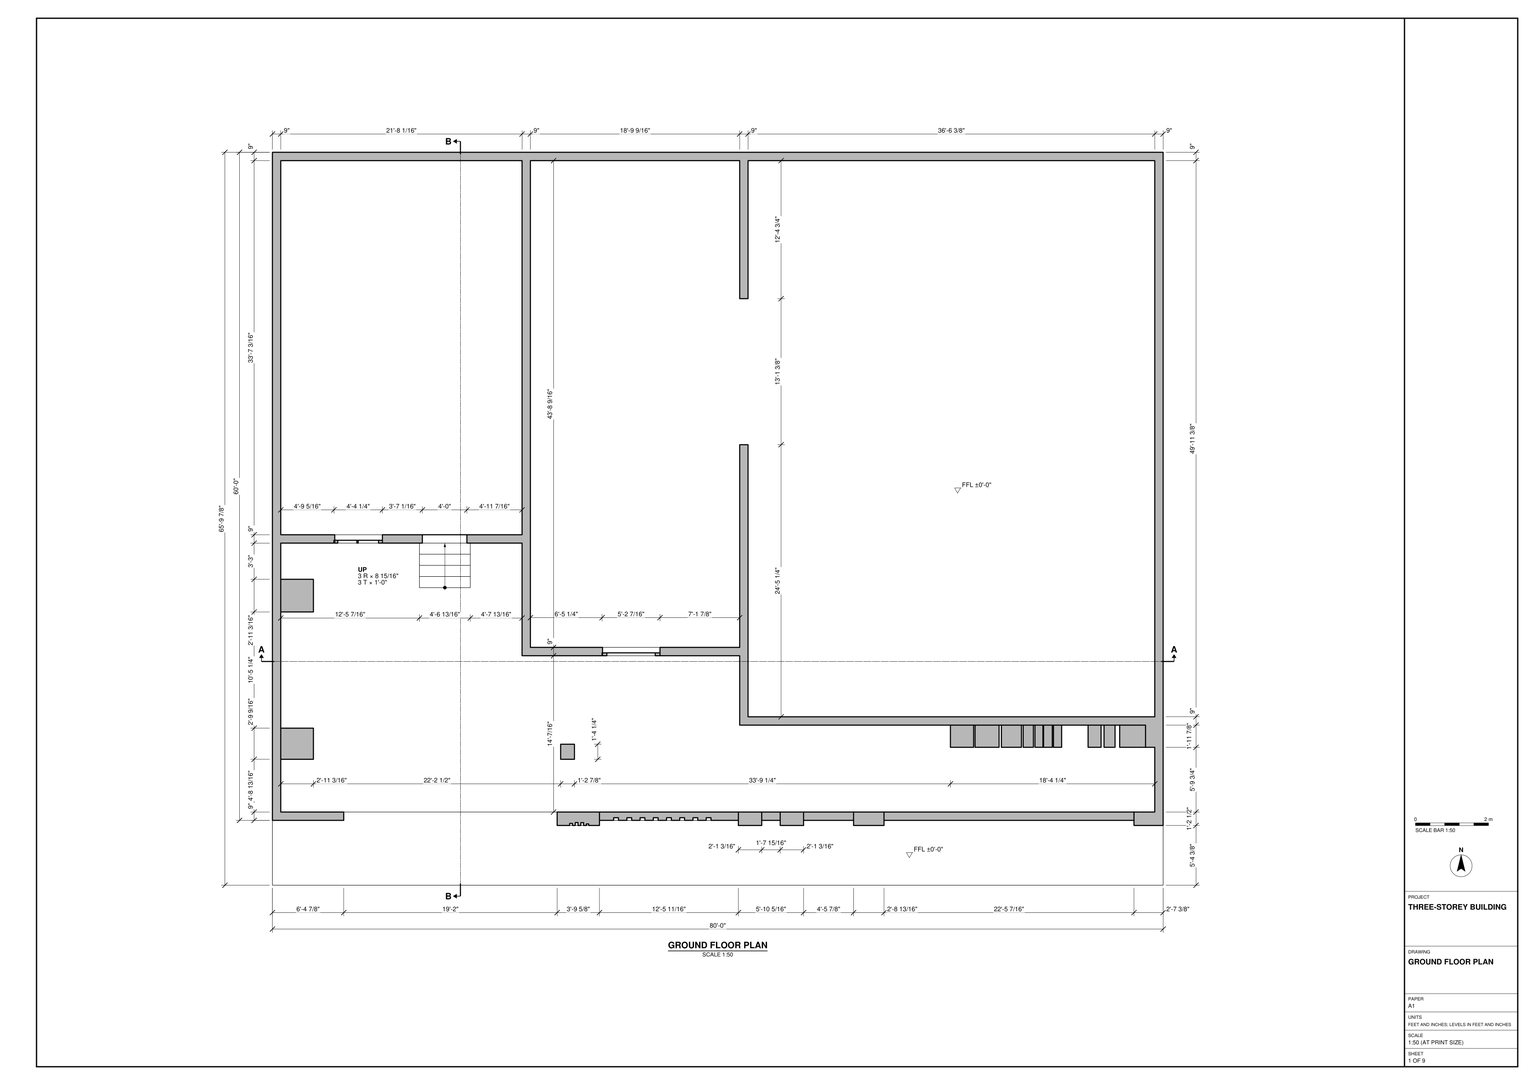
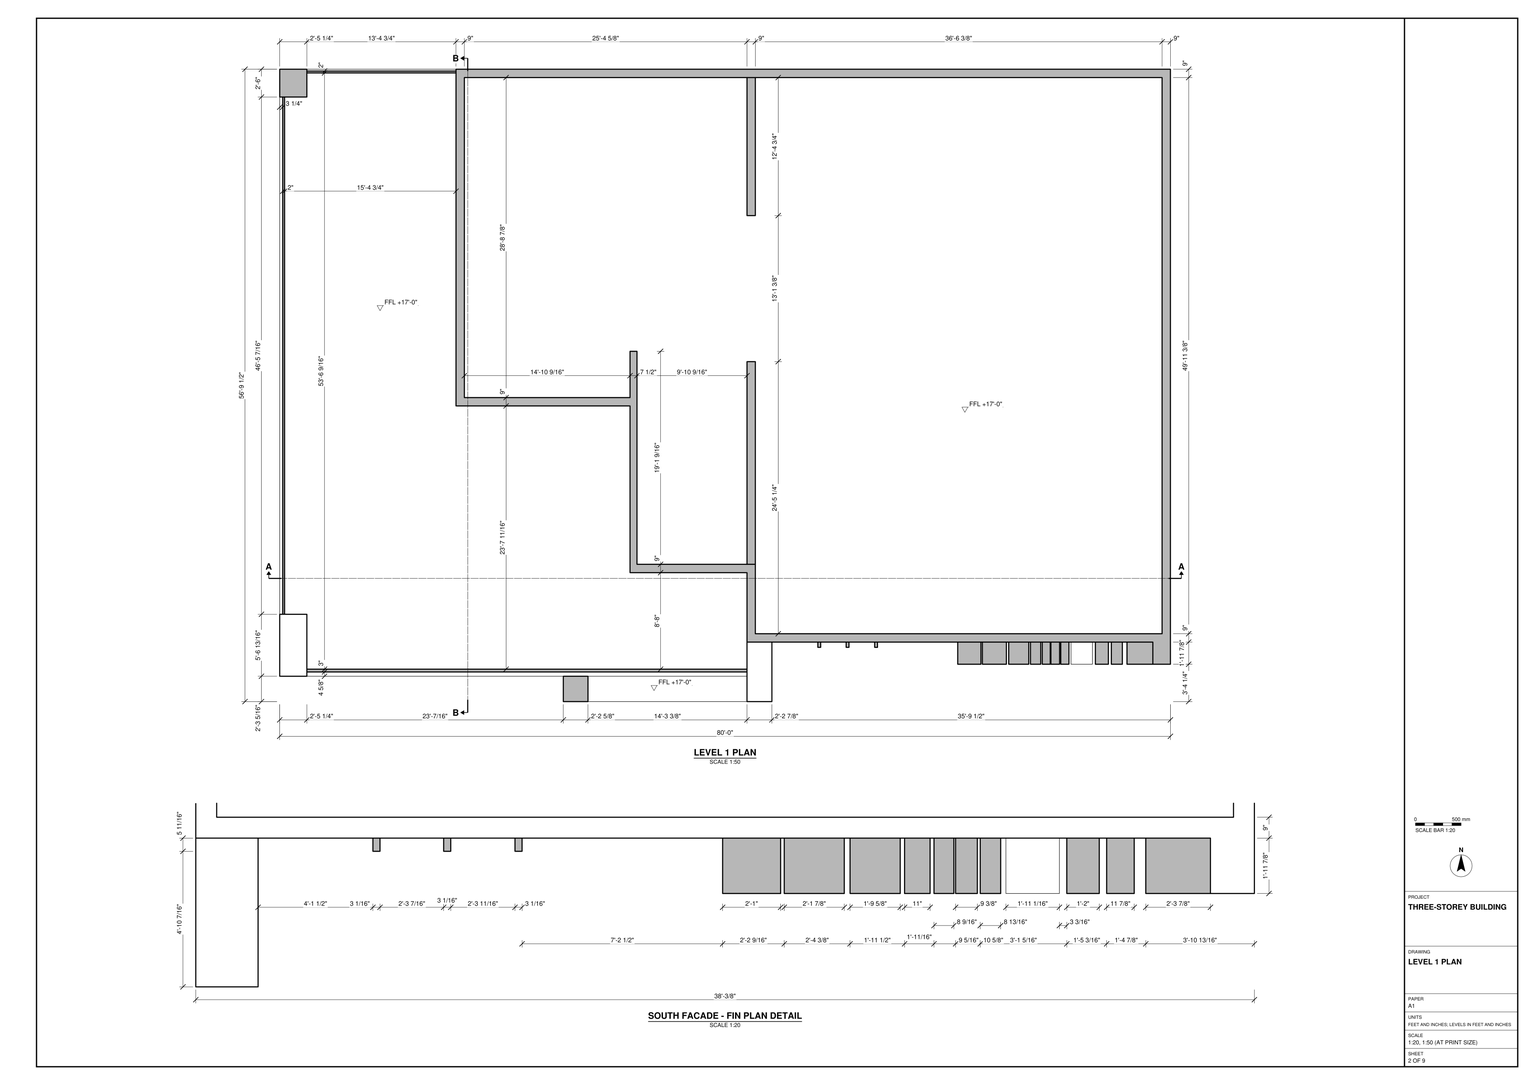
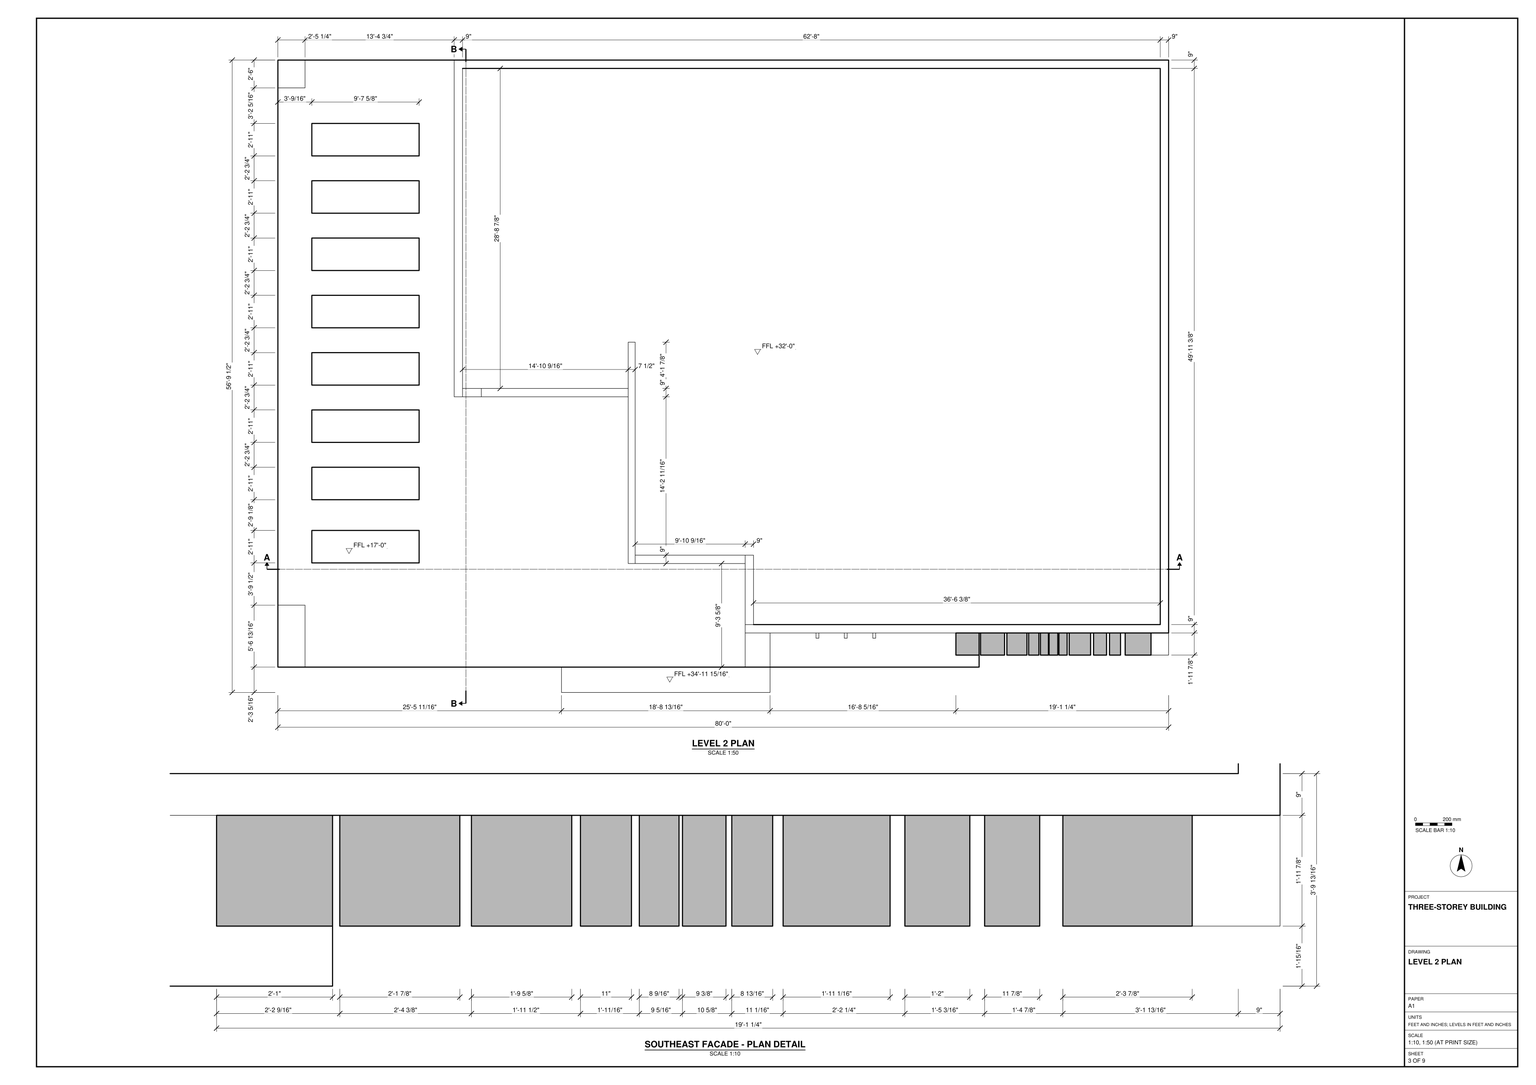
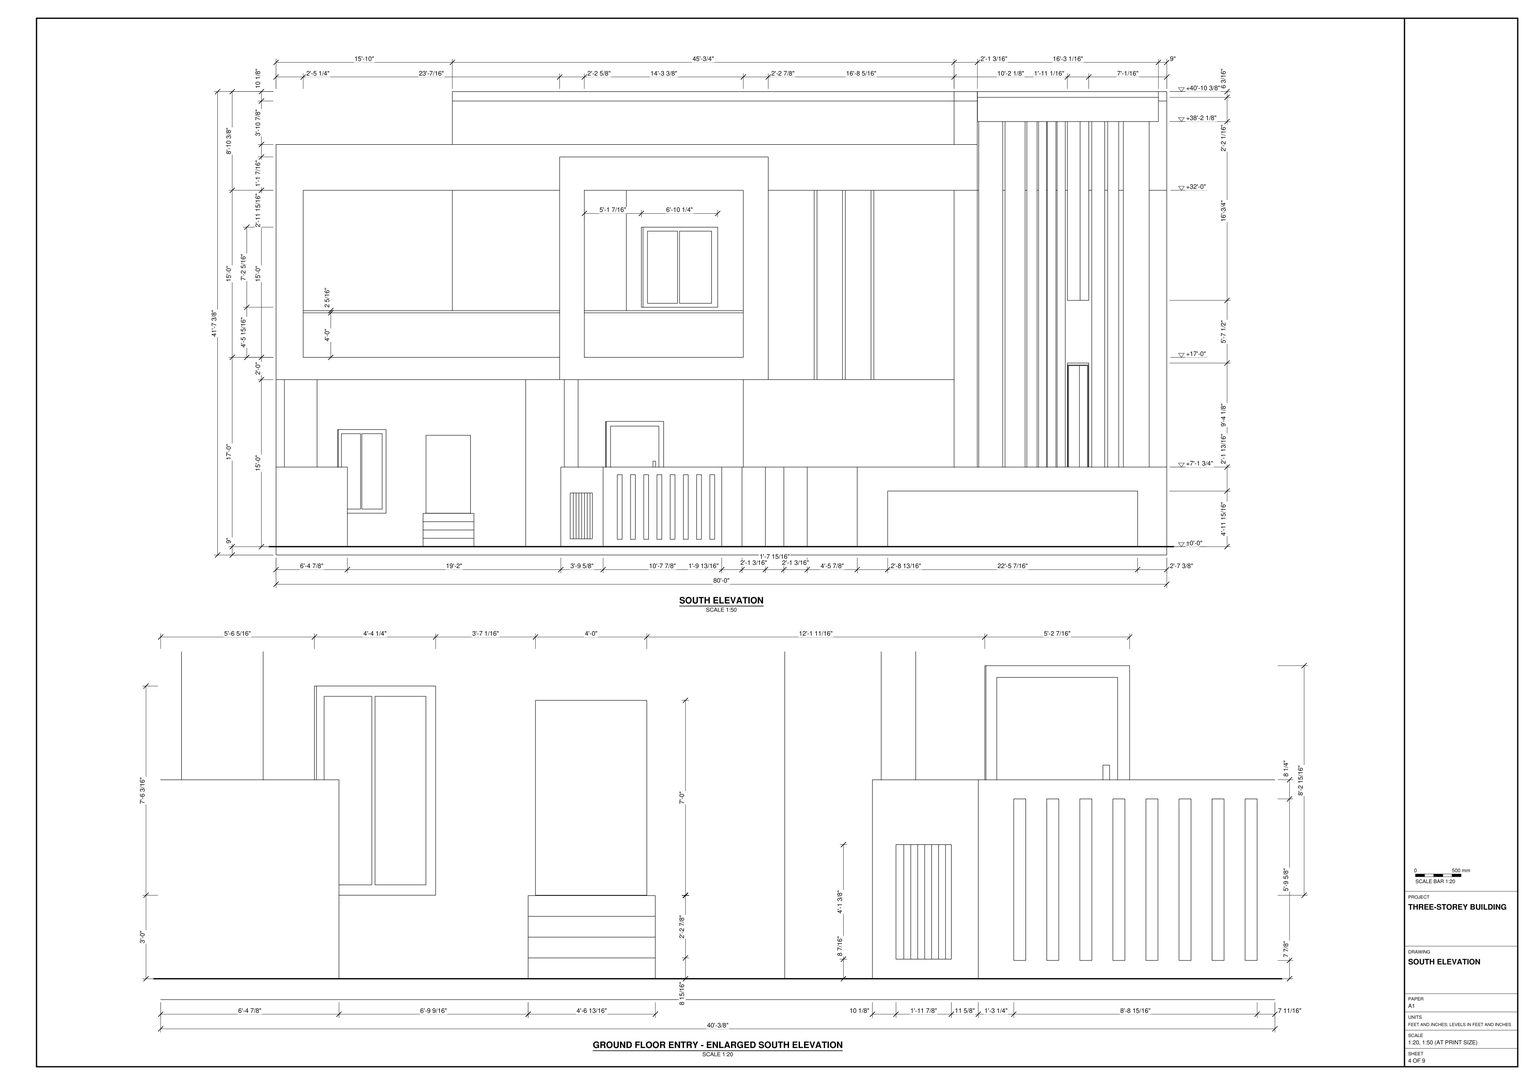
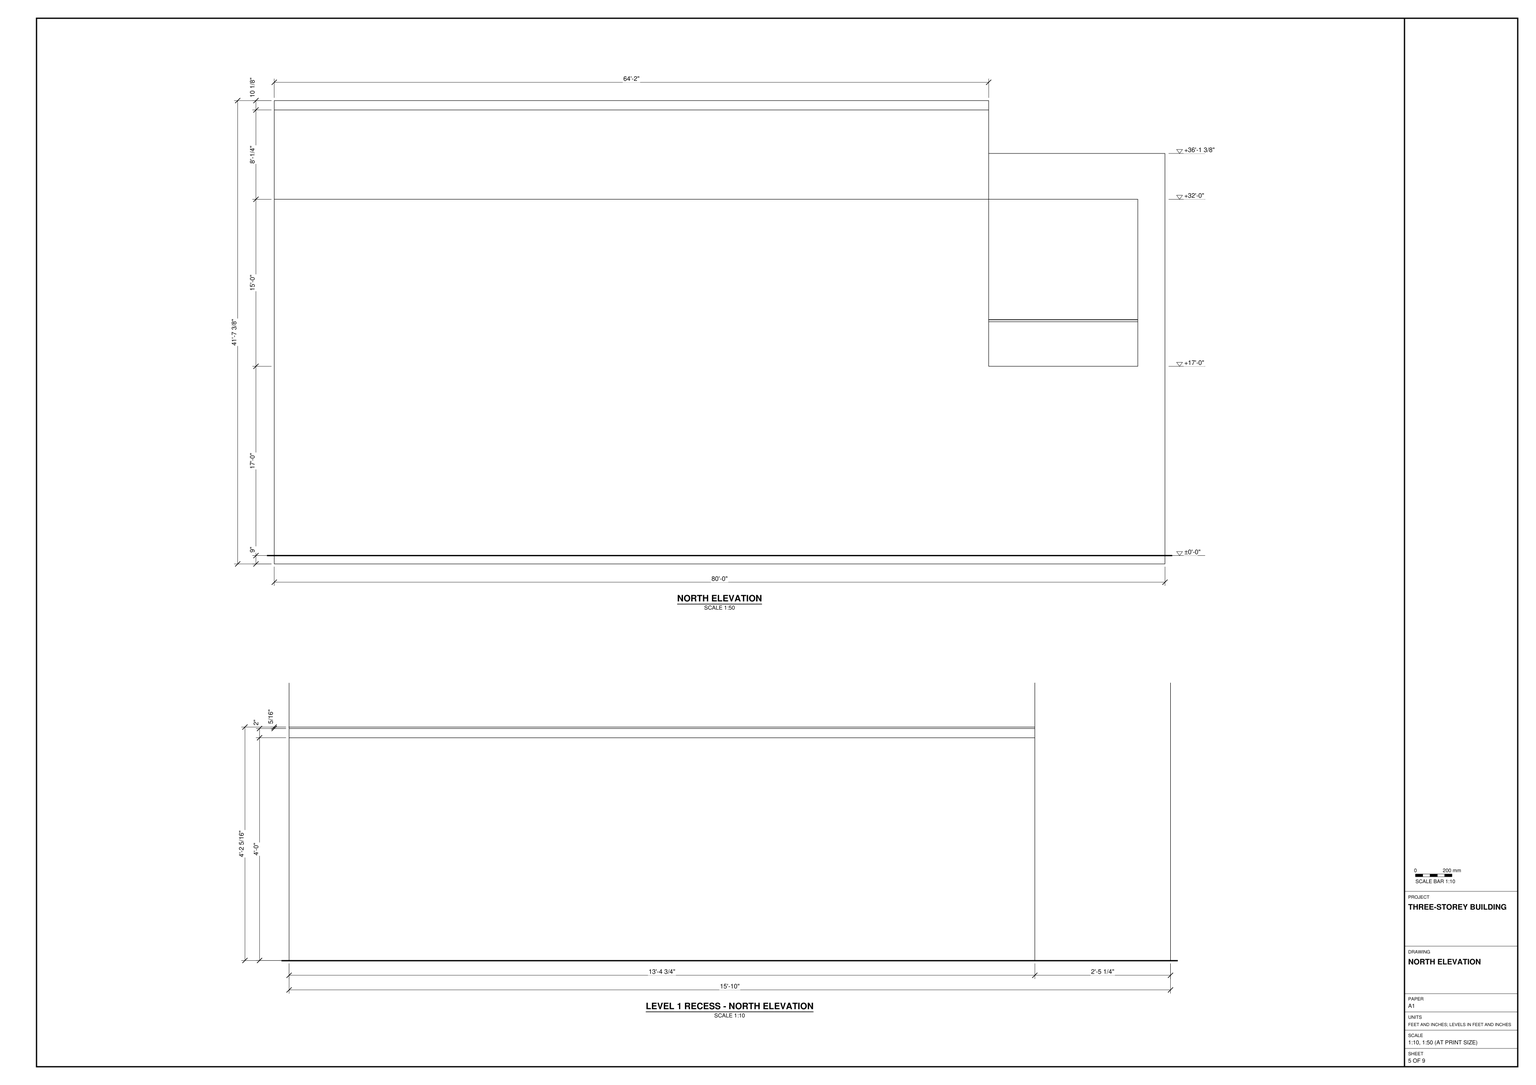
Build the three-storey building in SketchUp using task_files/diagram_01.pdf. Work in feet and inches. The overall model extents are 80'-0" east to west, 65'-9 7/8" north to south and 41'-7 3/8" vertically. Set the finished floor levels at ±0'-0", +17'-0" and +32'-0".

Lay out the ground floor from the north wall. The west, middle and east bays extend successively farther south, leaving an open area between the rooms and the south boundary wall. Follow the wall thicknesses shown, including the 9" walls. Form the door and window openings, the short stair at the south wall of the west room, and the wide entrance gap in the south boundary wall.

Follow each upper plan separately when modelling the walls, slabs and roof. Preserve the stepped enclosure and the terrace along its west and south sides. Use the upper plan to locate the row of rectangular openings above the west side. Model the projecting fins on the south face of the east bay, using the enlarged details for their widths and spacing.

Keep walls, slabs, roof, stairs and any furniture or joinery pieces shown in separate groups or components. Use components for repeated parts. Any decor or loose items shown may use suitable library components. Save one SketchUp model as output_files/three_storey_building_with_stepped_bays_and_facade_fins.skp.

# SketchUp Ruby script. Lengths in inches.
U = 1.inch
M = Sketchup.active_model
def pt(a) = Geom::Point3d.new(a.map { |v| v * U })
def face(e, loops, mat)
  f = e.add_face(loops[0].map { |a| pt(a) })
  loops[1..].each { |l| e.add_face(l.map { |a| pt(a) }).erase! }
  f.material = f.back_material = mat if mat
  f
end
# faces: each face lists its corners as indices into pts; further lists are holes
def faces(e, pts, list, mat = nil) = list.each { |f| face(e, (f[0].is_a?(Array) ? f : [f]).map { |l| l.map { |i| pts[i] } }, mat) }
# xy, xz, yz: faces in a plane at the given z, y or x. An outline is a flat list of corners, or four numbers for a rectangle; further outlines are holes
def ring(l) = l.size == 4 ? [[l[0], l[1]], [l[2], l[1]], [l[2], l[3]], [l[0], l[3]]] : l.each_slice(2).to_a
def flat(e, list, mat, &to3) = list.each { |f| face(e, (f[0].is_a?(Array) ? f : [f]).map { |l| ring(l).map { |u, v| to3.(u, v) } }, mat) }
def xy(e, z, list, mat = nil) = flat(e, list, mat) { |x, y| [x, y, z] }
def xz(e, y, list, mat = nil) = flat(e, list, mat) { |x, z| [x, y, z] }
def yz(e, x, list, mat = nil) = flat(e, list, mat) { |y, z| [x, y, z] }
def lines(e, pts, list) = list.each { |a, b| e.add_line(pt(pts[a]), pt(pts[b])) }
# prism: a flat outline (further loops are holes) pulled along v
def prism(e, loops, v, mat = nil)
  f = face(e, loops, mat); d = Geom::Vector3d.new(v.map { |x| x * U })
  f.pushpull(f.normal.samedirection?(d) ? d.length : -d.length)
end
def box(e, o, s, mat = nil) = prism(e, [[o, [o[0] + s[0], o[1], o[2]], [o[0] + s[0], o[1] + s[1], o[2]], [o[0], o[1] + s[1], o[2]]]], [0, 0, s[2]], mat)
def at(x, y, z, deg = 0) = Geom::Transformation.translation(pt([x, y, z])) * Geom::Transformation.rotation(ORIGIN, Z_AXIS, deg.degrees)
def axes(o, x, y, z) = Geom::Transformation.new([*x, 0, *y, 0, *z, 0, *pt(o).to_a, 1])
def part(name) = M.definitions.add(name)
# library, detail: a bought-in or finely detailed component or shape, given as its bounding box
def library(name, o, s) = part(name).tap { |d| box(d.entities, o, s) }
def detail(e, o, s) = box(e.add_group.entities, o, s)
def put(e, d, t, mat = nil) = e.add_instance(d, t).tap { |i| i.material = mat if mat }
def group(e, t, mat = nil) = e.add_group.tap { |g| g.transformation = t; g.material = mat if mat }.entities
root = M.entities
M.materials.add("[Carrera Marble]").color = [207, 207, 207]
M.materials.add("[Color B08]").color = [102, 25, 0]
M.materials.add("[Color C07]").color = [153, 76, 0]
M.materials.add("[Color C08]").color = [68, 51, 0]
M.materials.add("[Color C08]1").color = [76, 51, 0]
M.materials.add("[Color M00]").color = [255, 255, 255]
M.materials.add("[Color M03]").color = [170, 170, 170]
M.materials.add("[Color M04]").color = [142, 142, 142]
M.materials.add("[Color M06]").color = [86, 86, 86]
M.materials.add("[Metal Corrugated Shiny]").color = [193, 193, 193]
M.materials.add("[Sandstone]").color = [118, 81, 52]
M.materials.add("[Translucent Glass Gray]").color = [128, 128, 128]
M.materials["[Translucent Glass Gray]"].alpha = 0.5
M.materials.add("[Wood Bamboo]").color = [177, 105, 43]
c1 = part("Group\#2")
xy(c1.entities,0,[[0,0,104.5,6.125]],"[Translucent Glass Gray]")
xy(c1.entities,8.36,[[8.36,0,49.5,6.125],[52.25,0,96.14,6.125]],"[Color B08]")
xy(c1.entities,160.72,[[8.36,0,49.5,6.125],[52.25,0,96.14,6.125]],"[Color B08]")
xy(c1.entities,169.08,[[0,0,104.5,6.125]],"[Color B08]")
xz(c1.entities,0,[[[0,0,104.5,169.08],[52.25,8.36,96.14,160.72],[8.36,8.36,49.5,160.72]]],"[Color B08]")
xz(c1.entities,6.125,[[[0,0,104.5,169.08],[52.25,8.36,96.14,160.72],[8.36,8.36,49.5,160.72]]],"[Color B08]")
xz(c1.entities,6.125,[[8.36,8.36,49.5,160.72],[52.25,8.36,96.14,160.72]],"[Translucent Glass Gray]")
yz(c1.entities,0,[[0,0,6.125,169.08]],"[Color B08]")
yz(c1.entities,8.36,[[0,8.36,6.125,160.72]],"[Color B08]")
yz(c1.entities,49.5,[[0,8.36,6.125,160.72]],"[Color B08]")
yz(c1.entities,52.25,[[0,8.36,6.125,160.72]],"[Color B08]")
yz(c1.entities,96.14,[[0,8.36,6.125,160.72]],"[Color B08]")
yz(c1.entities,104.5,[[0,0,6.125,169.08]],"[Color B08]")
xy(root,0,[[0,0,960,789.875]])
xy(root,9,[[0,0,960,0,960,64.375,928.61,64.375,928.61,69.875,659.17,69.875,659.17,64.375,626.35,64.375,626.35,69.875,572.49,69.875,572.49,64.375,547.29,64.375,547.29,69.875,527.38,69.875,527.38,64.375,502.1875,64.375,502.1875,69.875,352.5,69.875,352.5,64.375,306.87,64.375,306.87,78.875,76.87,78.875,76.87,69.875,0,69.875],[306.87,64.375,352.5,78.875],[502.1875,64.375,527.38,78.875],[547.29,64.375,572.49,78.875],[626.35,64.375,659.17,78.875],
  [928.61,64.375,928.61,78.875,951,78.875,951,79.0625,960,79.0625,960,64.375],[0,69.875,0,368.6875,9,368.6875,9,78.875,76.87,78.875,76.87,69.875],[352.5,69.875,502.1875,78.875],[527.38,69.875,547.29,78.875],[572.49,69.875,626.35,78.875],
  [659.17,69.875,928.61,78.875],[[9,78.875,626.35,78.875,626.35,79.0625,659.17,79.0625,659.17,78.875,928.61,78.875,928.61,79.0625,951,79.0625,951,148.625,913.18,148.625,913.18,172.5,908.19,172.5,908.19,148.625,896.32,148.625,896.32,172.5,893.13,172.5,893.13,148.625,879.13,148.625,879.13,172.5,850.63,172.5,850.63,148.625,841.82,148.625,841.82,172.5,840.57,172.5,840.57,148.625,831.19,148.625,831.19,172.5,830.44,172.5,830.44,148.625,821.88,148.625,821.88,172.5,820.19,172.5,820.19,148.625,809.19,148.625,809.19,172.5,807.32,172.5,807.32,148.625,785.69,148.625,785.69,172.5,783.19,172.5,783.19,148.625,757.32,148.625,757.32,172.5,755.75,172.5,755.75,148.625,730.75,148.625,730.75,172.5,503.625,172.5,503.625,247.3125,269.0625,247.3125,269.0625,368.6875,213.25,368.6875,213.25,320.6875,158.44,320.6875,158.44,368.6875,9,368.6875,9,329.68,44.1875,329.68,44.1875,294.5,9,294.5,9,169.25,44.1875,169.25,44.1875,135.6875,9,135.6875],[310.66,135.6875,325.53,151.9375]],[626.35,78.875,659.17,79.0625],[928.61,78.875,951,79.0625],[951,79.0625,960,148.625],
  [730.75,148.625,755.75,172.5],[757.32,148.625,783.19,172.5],[785.69,148.625,807.32,172.5],[809.19,148.625,820.19,172.5],[821.88,148.625,830.44,172.5],
  [831.19,148.625,840.57,172.5],[841.82,148.625,850.63,172.5],[879.13,148.625,893.13,172.5],[896.32,148.625,908.19,172.5],[913.18,148.625,941.0625,172.5],
  [941.0625,148.625,960,172.5],[[503.625,172.5,503.625,247.3125,269.0625,247.3125,269.0625,368.6875,0,368.6875,0,789.875,960,789.875,960,172.5],[512.625,181.5,951,181.5,951,780.875,512.625,780.875,512.625,632.12,503.625,632.12,503.625,780.875,278.0625,780.875,278.0625,256.3125,503.625,256.3125,503.625,474.74,512.625,474.74],[9,377.6875,269.0625,780.875]],[512.625,181.5,951,181.5,951,780.875,512.625,780.875,512.625,632.12,503.625,632.12,503.625,780.875,278.0625,780.875,278.0625,256.3125,503.625,256.3125,503.625,474.74,512.625,474.74],[158.44,320.6875,213.25,332.6875],[158.44,332.6875,213.25,368.6875],
  [9,377.6875,269.0625,780.875]])
xy(root,9,[[9,135.6875,44.1875,169.25],[9,294.5,44.1875,329.68]],"[Color M06]")
xy(root,16.88,[[367.78,69.875,372.96,72.75],[382.03,69.875,387.21,72.75],[396.28,69.875,401.46,72.75],[410.53,69.875,415.71,72.75],[424.78,69.875,429.96,72.75],
  [439.03,69.875,444.21,72.75],[453.28,69.875,458.46,72.75],[467.53,69.875,472.71,72.75]],"[Color C08]1")
xy(root,17.43,[[320.38,64.375,323.38,66.625],[326.38,64.375,329.38,67.5625],[332.38,64.375,335.38,67.4375],[338.38,64.375,340.89,66.0625]],"[Sandstone]")
xy(root,17.96,[[158.44,320.6875,213.25,332.6875]])
xy(root,26.92,[[158.44,332.6875,213.25,344.6875]])
xy(root,35.88,[[158.44,344.6875,213.25,356.6875]])
xy(root,44.84,[[158.44,356.6875,213.25,368.6875]])
xy(root,45,[[355.8,247.3125,417.74,256.3125],[67.1875,368.6875,118.54,377.6875]])
xy(root,45,[[161.6,368.6875,209.6,377.6875]],"[Color B08]")
xy(root,66.8,[[320.38,64.375,323.38,66.625],[326.38,64.375,329.38,67.5625],[332.38,64.375,335.38,67.4375],[338.38,64.375,340.89,66.0625]],"[Sandstone]")
xy(root,68.92,[[659.17,64.375,928.61,69.875],[659.17,69.875,928.61,79.0625]],"[Color M06]")
xy(root,86.51,[[367.78,69.875,372.96,72.75],[382.03,69.875,387.21,72.75],[396.28,69.875,401.46,72.75],[410.53,69.875,415.71,72.75],[424.78,69.875,429.96,72.75],
  [439.03,69.875,444.21,72.75],[453.28,69.875,458.46,72.75],[467.53,69.875,472.71,72.75]],"[Color C08]1")
xy(root,94.75,[[0,69.875,76.87,69.875,76.87,78.875,9,78.875,9,368.6875,0,368.6875],[527.38,69.875,547.29,78.875],[572.49,69.875,626.35,78.875],[951,79.0625,960,148.625]])
xy(root,94.75,[[306.87,64.375,352.5,78.875]],"[Carrera Marble]")
xy(root,94.75,[[852.88,148.625,852.88,172.5,875.94,172.5,875.94,148.625,875.31,148.625,875.31,149.375,874.51,149.375,874.51,148.625,854.18,148.625,854.18,149.375,853.39,149.375,853.39,148.625]],"[Color C07]")
xy(root,94.75,[[352.5,69.875,480.37,78.875]],"[Color C08]1")
xy(root,94.75,[[480.37,69.875,502.1875,78.875]],"[Color M00]")
xy(root,94.75,[[502.1875,64.375,527.38,78.875],[547.29,64.375,572.49,78.875],[626.35,64.375,960,64.375,960,79.0625,951,79.0625,951,78.875,626.35,78.875],[626.35,78.875,951,79.0625]],"[Color M06]")
xy(root,129,[[161.6,368.6875,209.6,377.6875]],"[Color B08]")
xy(root,135.18,[[67.1875,368.6875,118.54,377.6875]])
xy(root,143.9375,[[355.8,247.3125,417.74,256.3125]])
xy(root,189,[[[0,135.6875,0,368.6875,269.0625,368.6875,269.0625,247.3125,503.625,247.3125,503.625,135.6875,325.53,135.6875,325.53,151.9375,310.66,151.9375,310.66,135.6875,44.1875,135.6875,44.1875,169.25,9,169.25,9,135.6875],[9,294.5,44.1875,329.68]],[579.99,166.8125,583.04,172.5],[610.49,166.8125,613.54,172.5],[641.24,166.8125,644.29,172.5]])
xy(root,189,[[503.625,135.6875,530.47,172.5]],"[Color M04]")
xy(root,189,[[305.66,108.375,530.47,135.6875],[9,135.6875,44.1875,169.25],[310.66,135.6875,325.53,151.9375]],"[Color M06]")
xy(root,204.07,[[865.88,148.625,874.51,149.375]],"[Color C07]")
xy(root,204.07,[[854.18,148.625,865.88,149.375]],"[Color C08]")
xy(root,204.77,[[853.39,148.625,875.31,149.375]],"[Color C08]")
xy(root,206.86,[[852.88,148.625,875.94,172.5]],"[Color C07]")
xy(root,207,[[512.625,181.5,512.625,474.74,503.625,474.74,503.625,256.3125,278.0625,256.3125,278.0625,780.875,503.625,780.875,503.625,632.12,512.625,632.12,512.625,780.875,951,780.875,951,181.5],[9,377.6875,269.0625,780.875]])
xy(root,213,[[29.25,135.6875,503.625,140.3125],[29.25,140.3125,503.625,143.3125],[29.25,143.3125,503.625,143.3125,503.625,247.3125,377.5625,247.3125,377.5625,427,190,427,190,785.875,29.25,785.875,29.25,759.9,5.25,759.9,5.25,202.47,29.25,202.47],[512.625,181.5,951,181.5,951,780.875,512.625,780.875,512.625,632.12,503.625,632.12,503.625,780.875,199,780.875,199,436,377.5625,436,377.5625,485.875,385.0625,485.875,385.0625,256.3125,503.625,256.3125,503.625,474.74,512.625,474.74],[0,202.47,3.25,759.9],
  [3.25,202.47,5.25,759.9],[503.625,256.3125,512.625,474.74],[503.625,632.12,512.625,780.875],[29.25,785.875,190,787.875],[29.25,787.875,190,789.875]])
xy(root,213,[[332.25,108.375,503.625,135.6875]],"[Color M06]")
xy(root,261,[[29.25,140.3125,503.625,143.3125],[3.25,202.47,5.25,759.9],[29.25,785.875,190,787.875]],"[Color B08]")
xy(root,263,[[3.25,202.47,5.25,759.9],[29.25,785.875,190,787.875]],"[Color B08]")
xy(root,263.3125,[[29.25,140.3125,503.625,143.3125]],"[Color B08]")
xy(root,266.95,[[395.49,247.3125,475.99,256.3125]])
xy(root,274.36,[[852.88,148.625,875.94,172.5]],"[Color C08]")
xy(root,353.26,[[395.49,247.3125,475.99,256.3125]])
xy(root,387,[[512.625,181.5,512.625,474.74,503.625,474.74,503.625,256.3125,385.0625,256.3125,385.0625,485.875,377.5625,485.875,377.5625,436,199,436,199,780.875,503.625,780.875,503.625,632.12,512.625,632.12,512.625,780.875,951,780.875,951,181.5]])
xy(root,393,[[503.625,135.6875,530.47,172.5],[530.47,135.6875,530.47,172.5,579.99,172.5,579.99,166.8125,583.04,166.8125,583.04,172.5,610.49,172.5,610.49,166.8125,613.54,166.8125,613.54,172.5,641.24,172.5,641.24,166.8125,644.29,166.8125,644.29,172.5,730.75,172.5,730.75,148.625,755.75,148.625,755.75,135.6875],[941.0625,148.625,960,172.5],[579.99,166.8125,583.04,172.5],[610.49,166.8125,613.54,172.5],
  [641.24,166.8125,644.29,172.5],[503.625,172.5,503.625,181.5,951,181.5,951,780.875,199,780.875,199,427,190,427,190,789.875,960,789.875,960,172.5],[512.625,181.5,951,181.5,951,780.875,199,780.875,199,436,377.5625,436,377.5625,485.875,385.0625,485.875,385.0625,256.3125,512.625,256.3125],[503.625,181.5,512.625,256.3125],[377.5625,247.3125,385.0625,485.875],
  [385.0625,247.3125,503.625,256.3125],[199,427,219.25,436],[219.25,427,377.5625,436]])
xy(root,393,[[[29.25,135.6875,503.625,135.6875,503.625,247.3125,377.5625,247.3125,377.5625,427,190,427,190,789.875,29.25,789.875,29.25,759.9,0,759.9,0,202.47,29.25,202.47],[36.58,247.98,152.21,282.98],[36.58,316.1,152.21,351.1],[36.58,377.85,152.21,412.85],[36.58,686.6,152.21,721.6],[36.58,624.85,152.21,659.85],[36.58,563.1,152.21,598.1],[36.58,501.35,152.21,536.35],[36.58,439.6,152.21,474.6]]],"[Color M00]")
xy(root,393,[[332.25,108.375,503.625,135.6875]],"[Color M06]")
xy(root,428.9375,[[305.66,108.375,530.47,135.6875]],"[Color M06]")
xy(root,442.375,[[[0,135.6875,755.75,135.6875,755.75,148.625,730.75,148.625,730.75,172.5,190,172.5,190,789.875,0,789.875],[36.58,686.6,152.21,721.6],[36.58,624.85,152.21,659.85],[36.58,563.1,152.21,598.1],[36.58,501.35,152.21,536.35],[36.58,439.6,152.21,474.6],[36.58,377.85,152.21,412.85],[36.58,316.1,152.21,351.1],[36.58,247.98,152.21,282.98]]],"[Color M00]")
xy(root,462.125,[[199,181.5,951,780.875]])
xy(root,467.125,[[755.96,172.5,951,181.5]])
xy(root,467.125,[[841.82,148.625,850.63,172.5],[879.13,148.625,893.13,172.5],[896.32,148.625,908.19,172.5]],"[Color C07]")
xy(root,467.125,[[757.32,148.625,783.19,172.5],[785.69,148.625,807.32,172.5],[809.19,148.625,820.19,172.5],[821.88,148.625,830.44,172.5],[831.19,148.625,840.57,172.5],
  [852.88,148.625,875.94,172.5],[913.18,148.625,941.0625,172.5]],"[Color C08]")
xy(root,467.125,[[755.96,126.9375,757.32,172.5],[757.32,126.9375,783.19,148.625],[783.19,126.9375,785.69,172.5],[785.69,126.9375,807.32,148.625],[807.32,126.9375,809.19,172.5],
  [809.19,126.9375,820.19,148.625],[820.19,126.9375,821.88,172.5],[821.88,126.9375,830.44,148.625],[830.44,126.9375,831.19,172.5],[831.19,126.9375,840.57,148.625],
  [840.57,126.9375,841.82,172.5],[841.82,126.9375,850.63,148.625],[850.63,126.9375,852.88,172.5],[852.88,126.9375,866.58,148.625],[866.58,126.9375,875.94,148.625],
  [875.94,126.9375,879.13,172.5],[879.13,126.9375,893.13,148.625],[893.13,126.9375,896.32,172.5],[896.32,126.9375,908.19,148.625],[908.19,126.9375,913.18,172.5],
  [913.18,126.9375,941.0625,148.625],[941.0625,126.9375,951,172.5],[199,181.5,755.96,181.5,755.96,442.33,951,442.33,951,780.875,199,780.875],[755.96,181.5,951,442.33]],"[Color M00]")
xy(root,489.25,[[730.75,148.625,755.75,172.5]],"[Color C08]")
xy(root,489.25,[[190,172.5,190,789.875,960,789.875,960,172.5,951,172.5,951,780.875,199,780.875,199,181.5,755.96,181.5,755.96,172.5]],"[Color M06]")
xy(root,493.1875,[[755.96,126.9375,951,442.33]],"[Color M00]")
xy(root,499.375,[[190,172.5,755.96,172.5,755.96,181.5,199,181.5,199,780.875,951,780.875,951,172.5,960,172.5,960,789.875,190,789.875]],"[Color M06]")
xz(root,0,[[0,0,960,9]])
xz(root,64.375,[[[306.87,9,352.5,94.75],[317.01,17.43,340.89,66.8]]],"[Carrera Marble]")
xz(root,64.375,[[502.1875,9,527.38,94.75],[547.29,9,572.49,94.75],[626.35,9,659.17,9,659.17,68.92,928.61,68.92,928.61,9,960,9,960,94.75,626.35,94.75]],"[Color M06]")
xz(root,64.375,[[317.01,17.43,320.38,66.8],[323.38,17.43,326.38,66.8],[329.38,17.43,332.38,66.8],[335.38,17.43,338.38,66.8]],"[Sandstone]")
xz(root,66.0625,[[338.38,17.43,340.89,66.8]],"[Sandstone]")
xz(root,66.625,[[320.38,17.43,323.38,66.8]],"[Sandstone]")
xz(root,67.4375,[[332.38,17.43,335.38,66.8]],"[Sandstone]")
xz(root,67.5625,[[326.38,17.43,329.38,66.8]],"[Sandstone]")
xz(root,69.875,[[0,9,76.87,94.75],[527.38,9,547.29,94.75],[572.49,9,626.35,94.75]])
xz(root,69.875,[[[352.5,9,480.37,94.75],[467.53,16.88,472.71,86.51],[453.28,16.88,458.46,86.51],[439.03,16.88,444.21,86.51],[424.78,16.88,429.96,86.51],[410.53,16.88,415.71,86.51],[396.28,16.88,401.46,86.51],[382.03,16.88,387.21,86.51],[367.78,16.88,372.96,86.51]]],"[Color C08]1")
xz(root,69.875,[[480.37,9,502.1875,94.75]],"[Color M00]")
xz(root,69.875,[[659.17,9,928.61,68.92]],"[Color M03]")
xz(root,72.75,[[367.78,16.88,372.96,86.51],[382.03,16.88,387.21,86.51],[396.28,16.88,401.46,86.51],[410.53,16.88,415.71,86.51],[424.78,16.88,429.96,86.51],
  [439.03,16.88,444.21,86.51],[453.28,16.88,458.46,86.51],[467.53,16.88,472.71,86.51]],"[Color C08]1")
xz(root,78.875,[[9,9,76.87,94.75],[527.38,9,547.29,94.75],[572.49,9,951,94.75]])
xz(root,78.875,[[306.87,9,352.5,94.75]],"[Carrera Marble]")
xz(root,78.875,[[352.5,9,480.37,94.75]],"[Color C08]1")
xz(root,78.875,[[480.37,9,502.1875,94.75]],"[Color M00]")
xz(root,78.875,[[502.1875,9,527.38,94.75],[547.29,9,572.49,94.75]],"[Color M06]")
xz(root,108.375,[[[305.66,189,530.47,428.9375],[332.25,213,503.625,393]]],"[Color M06]")
xz(root,126.9375,[[755.96,467.125,951,493.1875]],"[Color M00]")
xz(root,135.6875,[[305.66,189,332.25,213],[332.25,189,503.625,213],[305.66,213,332.25,393],[305.66,393,530.47,428.9375]])
xz(root,135.6875,[[0,189,305.66,189,305.66,213,29.25,213,29.25,393,305.66,393,305.66,428.9375,530.47,428.9375,530.47,393,755.75,393,755.75,442.375,0,442.375]],"[Color M00]")
xz(root,135.6875,[[9,9,44.1875,189],[310.66,9,325.53,189]],"[Color M06]")
xz(root,140.3125,[[29.25,261,503.625,263.3125]],"[Color B08]")
xz(root,140.3125,[[29.25,213,503.625,261]],"[Translucent Glass Gray]")
xz(root,143.3125,[[29.25,261,503.625,263.3125]],"[Color B08]")
xz(root,143.3125,[[29.25,213,503.625,261]],"[Translucent Glass Gray]")
xz(root,148.625,[[941.0625,9,951,9,951,94.75,960,94.75,960,393,941.0625,393],[730.75,393,755.75,442.375]])
xz(root,148.625,[[879.13,9,893.13,467.125],[896.32,9,908.19,467.125],[865.88,94.75,874.51,204.07],[866.58,274.36,875.94,467.125]],"[Color C07]")
xz(root,148.625,[[730.75,9,755.75,393],[757.32,9,783.19,467.125],[785.69,9,807.32,467.125],[809.19,9,820.19,467.125],[821.88,9,830.44,467.125],
  [831.19,9,840.57,467.125],[841.82,9,850.63,467.125],[913.18,9,941.0625,467.125],[852.88,94.75,853.39,94.75,853.39,204.77,875.31,204.77,875.31,94.75,875.94,94.75,875.94,206.86,852.88,206.86],[854.18,94.75,865.88,204.07],
  [852.88,274.36,866.58,467.125],[730.75,442.375,755.75,489.25]],"[Color C08]")
xz(root,149.375,[[853.39,94.75,854.18,94.75,854.18,204.07,874.51,204.07,874.51,94.75,875.31,94.75,875.31,204.77,853.39,204.77]],"[Color C08]")
xz(root,151.9375,[[310.66,9,325.53,189]],"[Color M06]")
xz(root,166.8125,[[579.99,189,583.04,393],[610.49,189,613.54,393],[641.24,189,644.29,393]])
xz(root,169.25,[[9,9,44.1875,189]],"[Color M06]")
xz(root,172.5,[[730.75,9,755.75,393],[757.32,9,783.19,393],[785.69,9,807.32,393],[809.19,9,820.19,393],[821.88,9,830.44,393],
  [831.19,9,840.57,393],[841.82,9,850.63,393],[879.13,9,893.13,393],[896.32,9,908.19,393],[913.18,9,941.0625,393],
  [852.88,94.75,875.94,206.86],[503.625,189,530.47,393],[579.99,189,583.04,393],[610.49,189,613.54,393],[641.24,189,644.29,393],
  [852.88,274.36,875.94,393],[730.75,393,755.75,489.25],[755.75,393,757.32,393,757.32,467.125,755.96,467.125,755.96,489.25,755.75,489.25],[757.32,393,783.19,467.125],[785.69,393,807.32,467.125],
  [809.19,393,820.19,467.125],[821.88,393,830.44,467.125],[830.44,393,831.19,467.125],[831.19,393,840.57,467.125],[840.57,393,841.82,467.125],
  [841.82,393,850.63,467.125],[852.88,393,875.94,467.125],[879.13,393,893.13,467.125],[896.32,393,908.19,467.125],[913.18,393,941.0625,467.125],
  [941.0625,393,960,393,960,489.25,951,489.25,951,467.125,941.0625,467.125]])
xz(root,172.5,[[[850.63,9,879.13,9,879.13,393,875.94,393,875.94,274.36,852.88,274.36,852.88,393,850.63,393],[852.88,94.75,875.94,206.86]],[893.13,9,896.32,393],[908.19,9,913.18,393],[850.63,393,852.88,467.125],[875.94,393,879.13,467.125],
  [893.13,393,896.32,467.125],[908.19,393,913.18,467.125]],"[Color C07]")
xz(root,172.5,[[755.75,9,757.32,393],[783.19,9,785.69,393],[807.32,9,809.19,393],[820.19,9,821.88,393],[830.44,9,831.19,393],
  [840.57,9,841.82,393],[783.19,393,785.69,467.125],[807.32,393,809.19,467.125],[820.19,393,821.88,467.125]],"[Color C08]")
xz(root,172.5,[[530.47,189,579.99,393],[583.04,189,610.49,393],[613.54,189,641.24,393],[644.29,189,730.75,393]],"[Color C08]1")
xz(root,172.5,[[503.625,9,730.75,189]],"[Color M00]")
xz(root,172.5,[[190,442.375,730.75,489.25]],"[Color M04]")
xz(root,172.5,[[190,489.25,730.75,499.375],[730.75,489.25,755.75,499.375],[755.75,489.25,755.96,499.375],[951,489.25,960,499.375]],"[Color M06]")
xz(root,181.5,[[512.625,9,951,189],[512.625,189,951,207],[512.625,207,523.6875,213],[523.6875,207,951,213],[512.625,213,523.6875,387],
  [523.6875,213,951,387],[512.625,387,523.6875,393],[523.6875,387,951,393],[512.625,393,951,462.125],[199,462.125,208.73,467.125],
  [208.73,462.125,217.42,467.125],[217.42,462.125,385.0625,467.125],[385.0625,462.125,512.625,467.125],[512.625,462.125,951,467.125],[199,467.125,755.96,489.25]])
xz(root,181.5,[[199,489.25,755.96,499.375]],"[Color M06]")
xz(root,202.47,[[0,213,0,393,29.25,393,29.25,213,5.25,213,5.25,263,3.25,263,3.25,213],[3.25,213,5.25,261]])
xz(root,202.47,[[3.25,261,5.25,263]],"[Color B08]")
xz(root,247.3125,[[[269.0625,9,503.625,189],[355.8,45,417.74,143.9375]]],"[Color M00]")
xz(root,247.3125,[[[377.5625,213,503.625,393],[395.49,266.95,475.99,353.26]]],"[Color M04]")
xz(root,247.98,[[36.58,393,152.21,442.375]],"[Color M00]")
xz(root,256.3125,[[[278.0625,9,503.625,189],[355.8,45,417.74,143.9375]],[278.0625,189,503.625,207],[[385.0625,213,503.625,387],[395.49,266.95,475.99,353.26]],[503.625,213,512.625,393],[385.0625,387,503.625,393]])
xz(root,282.98,[[36.58,393,152.21,442.375]],"[Color M00]")
xz(root,294.5,[[9,9,44.1875,189]],"[Color M06]")
xz(root,316.1,[[36.58,393,152.21,442.375]],"[Color M00]")
xz(root,320.6875,[[158.44,9,213.25,17.96]])
xz(root,329.68,[[9,9,44.1875,189]],"[Color M06]")
xz(root,332.6875,[[158.44,17.96,213.25,26.92]])
xz(root,344.6875,[[158.44,26.92,213.25,35.88]])
xz(root,351.1,[[36.58,393,152.21,442.375]],"[Color M00]")
xz(root,356.6875,[[158.44,35.88,213.25,44.84]])
xz(root,368.6875,[[[9,9,158.44,9,158.44,44.84,213.25,44.84,213.25,9,269.0625,9,269.0625,189,0,189,0,94.75,9,94.75],[67.1875,45,118.54,135.18],[161.6,45,209.6,129]],[158.44,9,213.25,35.88],[158.44,35.88,213.25,44.84]])
xz(root,377.6875,[[[9,9,269.0625,189],[67.1875,45,118.54,135.18],[161.6,45,209.6,129]],[9,189,269.0625,207]])
xz(root,377.6875,[[161.6,45,209.6,129]],"[Translucent Glass Gray]")
xz(root,377.85,[[36.58,393,152.21,442.375]],"[Color M00]")
xz(root,412.85,[[36.58,393,152.21,442.375]],"[Color M00]")
xz(root,427,[[190,213,377.5625,393]],"[Color M04]")
xz(root,436,[[199,213,377.5625,387],[199,387,219.25,393],[219.25,387,377.5625,393]])
xz(root,439.6,[[36.58,393,152.21,442.375]],"[Color M00]")
xz(root,442.33,[[755.96,467.125,951,493.1875]],"[Color M00]")
xz(root,474.6,[[36.58,393,152.21,442.375]],"[Color M00]")
xz(root,474.74,[[503.625,9,512.625,189],[503.625,189,512.625,207],[503.625,207,512.625,213],[503.625,213,512.625,387]])
xz(root,485.875,[[377.5625,213,385.0625,387],[377.5625,387,385.0625,393]])
xz(root,501.35,[[36.58,393,152.21,442.375]],"[Color M00]")
xz(root,536.35,[[36.58,393,152.21,442.375]],"[Color M00]")
xz(root,563.1,[[36.58,393,152.21,442.375]],"[Color M00]")
xz(root,598.1,[[36.58,393,152.21,442.375]],"[Color M00]")
xz(root,624.85,[[36.58,393,152.21,442.375]],"[Color M00]")
xz(root,632.12,[[503.625,9,512.625,189],[503.625,189,512.625,207],[503.625,207,512.625,213],[503.625,213,512.625,387]])
xz(root,659.85,[[36.58,393,152.21,442.375]],"[Color M00]")
xz(root,686.6,[[36.58,393,152.21,442.375]],"[Color M00]")
xz(root,721.6,[[36.58,393,152.21,442.375]],"[Color M00]")
xz(root,759.9,[[0,213,3.25,213,3.25,263,5.25,263,5.25,213,29.25,213,29.25,393,0,393],[3.25,213,5.25,261]])
xz(root,759.9,[[3.25,261,5.25,263]],"[Color B08]")
xz(root,780.875,[[9,9,269.0625,189],[278.0625,9,503.625,189],[512.625,9,951,189],[9,189,269.0625,207],[278.0625,189,503.625,207],
  [512.625,189,951,207],[278.0625,207,503.625,213],[512.625,207,951,213],[199,213,503.625,387],[503.625,213,512.625,393],
  [512.625,213,951,387],[199,387,503.625,393],[512.625,387,951,393],[199,393,951,462.125],[199,462.125,951,467.125],
  [199,467.125,951,489.25]])
xz(root,780.875,[[199,489.25,951,499.375]],"[Color M06]")
xz(root,785.875,[[29.25,261,190,263]],"[Color B08]")
xz(root,785.875,[[29.25,213,190,261]],"[Translucent Glass Gray]")
xz(root,787.875,[[29.25,261,190,263]],"[Color B08]")
xz(root,787.875,[[29.25,213,190,261]],"[Translucent Glass Gray]")
xz(root,789.875,[[0,0,960,9],[0,9,0,442.375,190,442.375,190,393,29.25,393,29.25,213,190,213,190,393,960,393,960,9]])
xz(root,789.875,[[190,393,960,489.25]],"[Color M04]")
xz(root,789.875,[[190,489.25,960,499.375]],"[Color M06]")
yz(root,0,[[0,0,789.875,9],[[69.875,9,69.875,94.75,368.6875,94.75,368.6875,189,135.6875,189,135.6875,442.375,789.875,442.375,789.875,9],[202.47,213,759.9,393]]])
yz(root,3.25,[[202.47,261,759.9,263]],"[Color B08]")
yz(root,3.25,[[202.47,213,759.9,261]],"[Translucent Glass Gray]")
yz(root,5.25,[[202.47,261,759.9,263]],"[Color B08]")
yz(root,5.25,[[202.47,213,759.9,261]],"[Translucent Glass Gray]")
yz(root,9,[[78.875,9,135.6875,94.75],[135.6875,9,169.25,94.75],[169.25,9,294.5,94.75],[294.5,9,329.68,94.75],[329.68,9,368.6875,94.75],
  [377.6875,9,780.875,189],[377.6875,189,780.875,207]])
yz(root,9,[[135.6875,94.75,169.25,189],[294.5,94.75,329.68,189]],"[Color M06]")
yz(root,29.25,[[135.6875,213,140.3125,213,140.3125,263.3125,143.3125,263.3125,143.3125,213,202.47,213,202.47,393,135.6875,393],[140.3125,213,143.3125,261],[759.9,213,785.875,213,785.875,263,787.875,263,787.875,213,789.875,213,789.875,393,759.9,393],[785.875,213,787.875,261]])
yz(root,29.25,[[140.3125,261,143.3125,263.3125],[785.875,261,787.875,263]],"[Color B08]")
yz(root,36.58,[[247.98,393,282.98,442.375],[316.1,393,351.1,442.375],[377.85,393,412.85,442.375],[439.6,393,474.6,442.375],[501.35,393,536.35,442.375],
  [563.1,393,598.1,442.375],[624.85,393,659.85,442.375],[686.6,393,721.6,442.375]],"[Color M00]")
yz(root,44.1875,[[135.6875,9,169.25,189],[294.5,9,329.68,189]],"[Color M06]")
yz(root,67.1875,[[368.6875,45,377.6875,135.18]])
yz(root,76.87,[[69.875,9,78.875,94.75]])
yz(root,118.54,[[368.6875,45,377.6875,135.18]])
yz(root,152.21,[[247.98,393,282.98,442.375],[316.1,393,351.1,442.375],[377.85,393,412.85,442.375],[439.6,393,474.6,442.375],[501.35,393,536.35,442.375],
  [563.1,393,598.1,442.375],[624.85,393,659.85,442.375],[686.6,393,721.6,442.375]],"[Color M00]")
yz(root,158.44,[[320.6875,9,320.6875,17.96,332.6875,17.96,332.6875,26.92,344.6875,26.92,344.6875,35.88,356.6875,35.88,356.6875,44.84,368.6875,44.84,368.6875,9]])
yz(root,161.6,[[368.6875,45,377.6875,129]],"[Color B08]")
yz(root,190,[[785.875,213,787.875,261]])
yz(root,190,[[785.875,261,787.875,263]],"[Color B08]")
yz(root,190,[[427,213,427,393,789.875,393,789.875,213,787.875,213,787.875,263,785.875,263,785.875,213],[172.5,442.375,780.875,489.25],[780.875,442.375,789.875,489.25]],"[Color M04]")
yz(root,190,[[172.5,489.25,780.875,499.375],[780.875,489.25,789.875,499.375]],"[Color M06]")
yz(root,199,[[436,213,780.875,387],[436,387,780.875,393],[181.5,462.125,780.875,467.125],[181.5,467.125,780.875,489.25]])
yz(root,199,[[181.5,489.25,780.875,499.375]],"[Color M06]")
yz(root,209.6,[[368.6875,45,377.6875,129]],"[Color B08]")
yz(root,213.25,[[320.6875,9,368.6875,9,368.6875,44.84,356.6875,44.84,356.6875,35.88,344.6875,35.88,344.6875,26.92,332.6875,26.92,332.6875,17.96,320.6875,17.96]])
yz(root,269.0625,[[247.3125,9,368.6875,189],[377.6875,9,780.875,189],[377.6875,189,780.875,207]])
yz(root,278.0625,[[256.3125,9,780.875,189],[256.3125,189,780.875,207]])
yz(root,305.66,[[108.375,189,135.6875,428.9375]],"[Color M06]")
yz(root,306.87,[[64.375,9,78.875,94.75]],"[Carrera Marble]")
yz(root,310.66,[[135.6875,9,151.9375,189]],"[Color M06]")
yz(root,320.38,[[64.375,17.43,66.625,66.8]],"[Sandstone]")
yz(root,323.38,[[64.375,17.43,66.625,66.8]],"[Sandstone]")
yz(root,325.53,[[135.6875,9,151.9375,189]],"[Color M06]")
yz(root,326.38,[[64.375,17.43,67.5625,66.8]],"[Sandstone]")
yz(root,329.38,[[64.375,17.43,67.5625,66.8]],"[Sandstone]")
yz(root,332.25,[[108.375,213,135.6875,393]],"[Color M06]")
yz(root,332.38,[[64.375,17.43,67.4375,66.8]],"[Sandstone]")
yz(root,335.38,[[64.375,17.43,67.4375,66.8]],"[Sandstone]")
yz(root,338.38,[[64.375,17.43,66.0625,66.8]],"[Sandstone]")
yz(root,340.89,[[64.375,17.43,66.0625,66.8]],"[Sandstone]")
yz(root,352.5,[[64.375,9,69.875,94.75],[69.875,9,78.875,94.75]])
yz(root,355.8,[[247.3125,45,256.3125,143.9375]])
yz(root,367.78,[[69.875,16.88,72.75,86.51]],"[Color C08]1")
yz(root,372.96,[[69.875,16.88,72.75,86.51]],"[Color C08]1")
yz(root,377.5625,[[436,213,485.875,387],[436,387,485.875,393]])
yz(root,377.5625,[[247.3125,213,427,393]],"[Color M04]")
yz(root,382.03,[[69.875,16.88,72.75,86.51]],"[Color C08]1")
yz(root,385.0625,[[256.3125,213,485.875,387],[256.3125,387,485.875,393]])
yz(root,387.21,[[69.875,16.88,72.75,86.51]],"[Color C08]1")
yz(root,395.49,[[247.3125,266.95,256.3125,353.26]])
yz(root,396.28,[[69.875,16.88,72.75,86.51]],"[Color C08]1")
yz(root,401.46,[[69.875,16.88,72.75,86.51]],"[Color C08]1")
yz(root,410.53,[[69.875,16.88,72.75,86.51]],"[Color C08]1")
yz(root,415.71,[[69.875,16.88,72.75,86.51]],"[Color C08]1")
yz(root,417.74,[[247.3125,45,256.3125,143.9375]])
yz(root,424.78,[[69.875,16.88,72.75,86.51]],"[Color C08]1")
yz(root,429.96,[[69.875,16.88,72.75,86.51]],"[Color C08]1")
yz(root,439.03,[[69.875,16.88,72.75,86.51]],"[Color C08]1")
yz(root,444.21,[[69.875,16.88,72.75,86.51]],"[Color C08]1")
yz(root,453.28,[[69.875,16.88,72.75,86.51]],"[Color C08]1")
yz(root,458.46,[[69.875,16.88,72.75,86.51]],"[Color C08]1")
yz(root,467.53,[[69.875,16.88,72.75,86.51]],"[Color C08]1")
yz(root,472.71,[[69.875,16.88,72.75,86.51]],"[Color C08]1")
yz(root,475.99,[[247.3125,266.95,256.3125,353.26]])
yz(root,502.1875,[[64.375,9,69.875,94.75],[69.875,9,78.875,94.75]],"[Color M06]")
yz(root,503.625,[[172.5,9,247.3125,189],[256.3125,9,474.74,189],[632.12,9,780.875,189],[135.6875,189,172.5,213],[172.5,189,247.3125,213],
  [256.3125,189,474.74,207],[632.12,189,780.875,207],[256.3125,207,474.74,213],[632.12,207,780.875,213],[140.3125,213,143.3125,261],
  [256.3125,213,474.74,387],[632.12,213,780.875,387]])
yz(root,503.625,[[140.3125,261,143.3125,263.3125]],"[Color B08]")
yz(root,503.625,[[172.5,213,247.3125,393]],"[Color M04]")
yz(root,503.625,[[108.375,213,108.375,393,172.5,393,172.5,213,143.3125,213,143.3125,263.3125,140.3125,263.3125,140.3125,213]],"[Color M06]")
yz(root,512.625,[[181.5,9,474.74,189],[632.12,9,780.875,189],[181.5,189,474.74,207],[632.12,189,780.875,207],[181.5,207,474.74,213],
  [632.12,207,780.875,213],[181.5,213,256.3125,387],[256.3125,213,474.74,387],[632.12,213,780.875,387],[181.5,387,256.3125,393]])
yz(root,527.38,[[64.375,9,69.875,94.75],[69.875,9,78.875,94.75]],"[Color M06]")
yz(root,530.47,[[108.375,189,172.5,393],[108.375,393,135.6875,428.9375]],"[Color M06]")
yz(root,547.29,[[64.375,9,69.875,94.75],[69.875,9,78.875,94.75]],"[Color M06]")
yz(root,572.49,[[64.375,9,69.875,94.75],[69.875,9,78.875,94.75]],"[Color M06]")
yz(root,579.99,[[166.8125,189,172.5,393]])
yz(root,583.04,[[166.8125,189,172.5,393]])
yz(root,610.49,[[166.8125,189,172.5,393]])
yz(root,613.54,[[166.8125,189,172.5,393]])
yz(root,626.35,[[64.375,9,69.875,94.75],[69.875,9,79.0625,94.75]],"[Color M06]")
yz(root,641.24,[[166.8125,189,172.5,393]])
yz(root,644.29,[[166.8125,189,172.5,393]])
yz(root,659.17,[[64.375,9,69.875,68.92],[69.875,9,79.0625,68.92]],"[Color M06]")
yz(root,730.75,[[148.625,393,172.5,442.375]])
yz(root,730.75,[[148.625,9,172.5,393],[148.625,442.375,172.5,489.25]],"[Color C08]")
yz(root,755.75,[[135.6875,393,148.625,442.375]])
yz(root,755.75,[[148.625,9,172.5,393],[148.625,393,172.5,489.25]],"[Color C08]")
yz(root,755.96,[[172.5,467.125,181.5,489.25]])
yz(root,755.96,[[126.9375,467.125,172.5,493.1875],[181.5,467.125,442.33,493.1875],[172.5,489.25,181.5,493.1875]],"[Color M00]")
yz(root,755.96,[[172.5,493.1875,181.5,499.375]],"[Color M06]")
yz(root,757.32,[[148.625,9,172.5,467.125]],"[Color C08]")
yz(root,783.19,[[148.625,9,172.5,393],[148.625,393,172.5,467.125]],"[Color C08]")
yz(root,785.69,[[148.625,9,172.5,467.125]],"[Color C08]")
yz(root,807.32,[[148.625,9,172.5,393],[148.625,393,172.5,467.125]],"[Color C08]")
yz(root,809.19,[[148.625,9,172.5,467.125]],"[Color C08]")
yz(root,820.19,[[148.625,9,172.5,393],[148.625,393,172.5,467.125]],"[Color C08]")
yz(root,821.88,[[148.625,9,172.5,467.125]],"[Color C08]")
yz(root,830.44,[[148.625,9,172.5,393],[148.625,393,172.5,467.125]],"[Color C08]")
yz(root,831.19,[[148.625,9,172.5,467.125]],"[Color C08]")
yz(root,840.57,[[148.625,9,172.5,393],[148.625,393,172.5,467.125]],"[Color C08]")
yz(root,841.82,[[148.625,9,172.5,467.125]],"[Color C07]")
yz(root,850.63,[[148.625,9,172.5,393],[148.625,393,172.5,467.125]],"[Color C07]")
yz(root,852.88,[[148.625,274.36,172.5,467.125]])
yz(root,852.88,[[148.625,94.75,172.5,206.86]],"[Color C08]")
yz(root,853.39,[[148.625,94.75,149.375,204.77]],"[Color C08]")
yz(root,854.18,[[148.625,94.75,149.375,204.07]],"[Color C08]")
yz(root,874.51,[[148.625,94.75,149.375,204.07]],"[Color C07]")
yz(root,875.31,[[148.625,94.75,149.375,204.77]],"[Color C08]")
yz(root,875.94,[[148.625,94.75,172.5,206.86],[148.625,274.36,172.5,467.125]],"[Color C07]")
yz(root,879.13,[[148.625,9,172.5,467.125]],"[Color C07]")
yz(root,893.13,[[148.625,9,172.5,467.125]],"[Color C07]")
yz(root,896.32,[[148.625,9,172.5,467.125]],"[Color C07]")
yz(root,908.19,[[148.625,9,172.5,467.125]],"[Color C07]")
yz(root,913.18,[[148.625,9,172.5,467.125]],"[Color C08]")
yz(root,928.61,[[64.375,9,69.875,68.92],[69.875,9,79.0625,68.92]],"[Color M06]")
yz(root,941.0625,[[148.625,9,172.5,393]])
yz(root,941.0625,[[148.625,393,172.5,467.125]],"[Color C08]")
yz(root,951,[[78.875,9,148.625,94.75],[181.5,9,780.875,189],[181.5,189,780.875,207],[181.5,207,780.875,213],[181.5,213,780.875,387],
  [181.5,387,780.875,393],[181.5,393,780.875,462.125],[181.5,462.125,780.875,467.125],[181.5,467.125,442.33,489.25],[442.33,467.125,780.875,489.25]])
yz(root,951,[[126.9375,467.125,172.5,493.1875],[172.5,467.125,181.5,489.25],[172.5,489.25,181.5,493.1875],[181.5,489.25,442.33,493.1875]],"[Color M00]")
yz(root,951,[[442.33,489.25,780.875,499.375],[172.5,493.1875,181.5,499.375],[181.5,493.1875,442.33,499.375]],"[Color M06]")
yz(root,960,[[0,0,789.875,9],[64.375,9,789.875,9,789.875,393,148.625,393,148.625,94.75,64.375,94.75]])
yz(root,960,[[172.5,393,789.875,489.25]],"[Color M04]")
yz(root,960,[[172.5,489.25,789.875,499.375]],"[Color M06]")
p = [[269.0625,780.875,207],[269.0625,780.875,213],[9,780.875,207],[9,780.875,213],[9,377.6875,207],[9,377.6875,213],
  [377.5625,436,213],[385.0625,436,213],[512.625,632.12,387],[512.625,632.12,393],[503.625,632.12,387],[503.625,632.12,393],
  [199,181.5,393],[199,181.5,462.125],[385.0625,181.5,393],[385.0625,181.5,462.125]]
lines(root,p,[[0,1],[2,3],[4,5],[6,7],[8,9],[10,11],[12,13],[14,15]])
g1 = group(root,at(355.32,247.3125,45))
xy(g1,0,[[0,0,62.42,3.09]],"[Wood Bamboo]")
xy(g1,5.04,[[5.15,0,57.27,3.09]],"[Wood Bamboo]")
xy(g1,35.19,[[50.93,1.65,53.8,3.09]],"[Metal Corrugated Shiny]")
xy(g1,56.08,[[50.93,1.65,53.8,3.09]],"[Metal Corrugated Shiny]")
xy(g1,93.89,[[5.15,0,57.27,3.09]],"[Wood Bamboo]")
xy(g1,98.9375,[[0,0,62.42,3.09]],"[Wood Bamboo]")
xz(g1,0,[[[0,0,62.42,98.9375],[5.15,5.04,57.27,93.89]]],"[Wood Bamboo]")
xz(g1,1.65,[[50.93,35.19,53.8,56.08]],"[Metal Corrugated Shiny]")
xz(g1,3.09,[[[0,0,62.42,98.9375],[5.15,5.04,57.27,93.89]],[[5.15,5.04,57.27,93.89],[50.93,35.19,53.8,56.08]],[50.93,35.19,53.8,56.08]],"[Wood Bamboo]")
yz(g1,0,[[0,0,3.09,98.9375]],"[Wood Bamboo]")
yz(g1,5.15,[[0,5.04,3.09,93.89]],"[Wood Bamboo]")
yz(g1,50.93,[[1.65,35.19,3.09,56.08]],"[Metal Corrugated Shiny]")
yz(g1,53.8,[[1.65,35.19,3.09,56.08]],"[Metal Corrugated Shiny]")
yz(g1,57.27,[[0,5.04,3.09,93.89]],"[Wood Bamboo]")
yz(g1,62.42,[[0,0,3.09,98.9375]],"[Wood Bamboo]")
put(root,c1,axes([66.29,368.6875,45],[0.5,0,0],[0,0.5,0],[0,0,0.53335]))
put(root,c1,axes([393.72,247.56,266.95],[0.78729,0,0],[0,0.46,0],[0,0,0.51047]))
